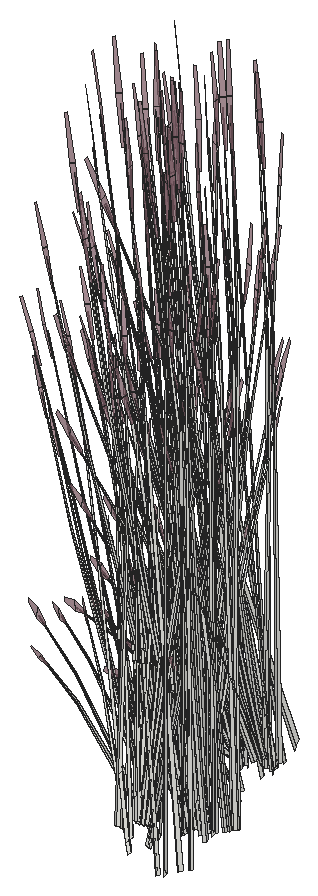
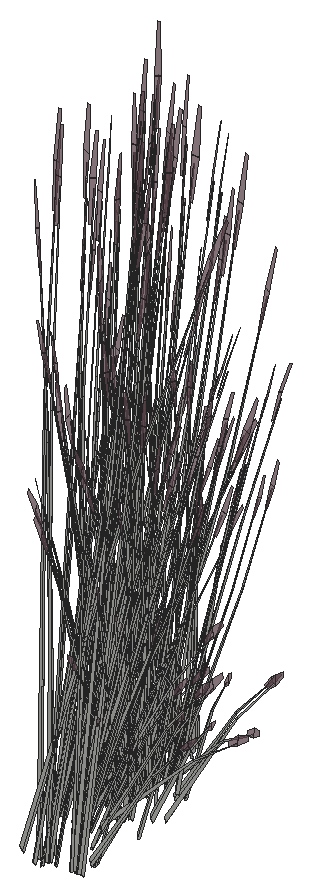
# SketchUp Ruby script. Lengths in inches.
U = 1.inch
M = Sketchup.active_model
def pt(a) = Geom::Point3d.new(a.map { |v| v * U })
def face(e, loops, mat)
  f = e.add_face(loops[0].map { |a| pt(a) })
  loops[1..].each { |l| e.add_face(l.map { |a| pt(a) }).erase! }
  f.material = f.back_material = mat if mat
  f
end
# faces: each face lists its corners as indices into pts; further lists are holes
def faces(e, pts, list, mat = nil) = list.each { |f| face(e, (f[0].is_a?(Array) ? f : [f]).map { |l| l.map { |i| pts[i] } }, mat) }
# xy, xz, yz: faces in a plane at the given z, y or x. An outline is a flat list of corners, or four numbers for a rectangle; further outlines are holes
def ring(l) = l.size == 4 ? [[l[0], l[1]], [l[2], l[1]], [l[2], l[3]], [l[0], l[3]]] : l.each_slice(2).to_a
def flat(e, list, mat, &to3) = list.each { |f| face(e, (f[0].is_a?(Array) ? f : [f]).map { |l| ring(l).map { |u, v| to3.(u, v) } }, mat) }
def xy(e, z, list, mat = nil) = flat(e, list, mat) { |x, y| [x, y, z] }
def xz(e, y, list, mat = nil) = flat(e, list, mat) { |x, z| [x, y, z] }
def yz(e, x, list, mat = nil) = flat(e, list, mat) { |y, z| [x, y, z] }
def lines(e, pts, list) = list.each { |a, b| e.add_line(pt(pts[a]), pt(pts[b])) }
# prism: a flat outline (further loops are holes) pulled along v
def prism(e, loops, v, mat = nil)
  f = face(e, loops, mat); d = Geom::Vector3d.new(v.map { |x| x * U })
  f.pushpull(f.normal.samedirection?(d) ? d.length : -d.length)
end
def box(e, o, s, mat = nil) = prism(e, [[o, [o[0] + s[0], o[1], o[2]], [o[0] + s[0], o[1] + s[1], o[2]], [o[0], o[1] + s[1], o[2]]]], [0, 0, s[2]], mat)
def at(x, y, z, deg = 0) = Geom::Transformation.translation(pt([x, y, z])) * Geom::Transformation.rotation(ORIGIN, Z_AXIS, deg.degrees)
def axes(o, x, y, z) = Geom::Transformation.new([*x, 0, *y, 0, *z, 0, *pt(o).to_a, 1])
def part(name) = M.definitions.add(name)
# library, detail: a bought-in or finely detailed component or shape, given as its bounding box
def library(name, o, s) = part(name).tap { |d| box(d.entities, o, s) }
def detail(e, o, s) = box(e.add_group.entities, o, s)
def put(e, d, t, mat = nil) = e.add_instance(d, t).tap { |i| i.material = mat if mat }
def group(e, t, mat = nil) = e.add_group.tap { |g| g.transformation = t; g.material = mat if mat }.entities
root = M.entities
M.materials.add("LightPink_Translucent").color = [144, 107, 117]
M.materials["LightPink_Translucent"].alpha = 0.75
c1 = part("blade")
p = [[2.15,0.21,22],[0,0.17,0],[0.09,0.45,0],[2.18,0.31,22],[2.29,0.31,22],[0.38,0.45,0],
  [2.48,0.24,33],[2.49,0.24,33],[2.48,0.22,33]]
faces(c1.entities,p,[[0,1,2,3],[4,5,2,3],[6,3,4,7],[8,0,3,6]])
c2 = part("seeds")
p = [[0.3,-0.1,1.38],[-0.01,-0.03,1.59],[-0.01,-0.03,0.03],[0.14,-0.07,-0.07],[0.29,-0.03,3],[0.15,0.01,3.11]]
faces(c2.entities,p,[[0,1,2,3],[1,0,4,5]],"LightPink_Translucent")
c3 = part("blade with seeds")
put(c3.entities,c1,at(0,0,0))
put(c3.entities,c2,axes([2.4,0.25,30.99],[1.5799,-0.05474,1.17369],[-0.12525,1.92788,0.29478],[-0.07173,-0.02425,1.56792]))
put(root,c3,axes([684.71,328.74,393.91],[0.04823,0.05698,1.47228],[-0.23252,0.51221,-0.13912],[-0.23548,0.00371,0.26054]))
put(root,c3,axes([685.2,321.78,393.91],[-0.10624,0.07413,1.45204],[0.00904,0.54162,-0.22964],[-0.24352,0.07044,0.11645]))
put(root,c3,axes([685.25,328.4,393.91],[-0.13998,-0.00403,1.45204],[-0.44565,0.40302,-0.22964],[-0.23779,-0.08235,0.11645]))
put(root,c3,axes([685.625,329.4,394.18],[-0.03484,0.58066,-0.10093],[-0.65957,-0.01587,-0.56021],[-0.25402,-0.04034,0.85122]))
put(root,c3,axes([685.54,321.47,393.76],[-0.54068,-0.15928,-0.29394],[0.1577,-0.46469,0.37948],[-0.21769,0.04261,0.72609]))
put(root,c3,axes([685.2,329.45,393.76],[-0.37017,-0.35748,-0.29394],[0.42268,-0.3384,0.37948],[-0.21476,-0.05149,0.72609]))
put(root,c3,axes([684.02,322.33,393.91],[0.08303,0.01531,1.47228],[0.25685,0.50448,-0.13912],[-0.16996,0.13241,0.26054]))
put(root,c3,axes([685.91,321.71,393.89],[-0.17625,0.51936,-0.42412],[-0.60429,-0.17802,-0.32852],[-0.2433,0.04762,0.81151]))
put(root,c3,axes([684.31,330.3,392.3],[0.41536,-0.04086,0.95334],[-0.26347,0.35999,0.70045],[-0.20525,-0.054,0.20998]))
put(root,c3,axes([685.61,321.68,391.24],[0.0165,0.08998,1.46364],[-0.33262,0.46992,-0.2236],[-0.23626,-0.02369,0.24931]))
put(root,c3,axes([685.14,329.3125,394.23],[0.53728,-0.42137,0.44623],[0.46337,0.44748,0.36794],[-0.25207,-0.07773,0.92337]))
put(root,c3,axes([684.72,323.93,392.3],[0.27113,-0.25877,0.95334],[0.10699,0.40966,0.70045],[-0.19594,0.07335,0.20998]))
put(root,c3,axes([685.67,321.41,393.93],[0.18381,-0.5206,0.39842],[0.60429,0.17802,0.32852],[-0.23764,0.03129,0.82444]))
put(root,c3,axes([685.88,321.26,394.18],[0.32734,0.51701,-0.10093],[-0.58097,0.25407,-0.56021],[-0.24483,0.06821,0.85122]))
put(root,c3,axes([686.62,320.19,394.18],[-0.03484,0.58066,-0.10093],[-0.65957,-0.01587,-0.56021],[-0.25402,-0.04034,0.85122]))
put(root,c3,axes([685.62,321.28,393.93],[-0.23895,-0.38931,0.05337],[0.43573,-0.19055,0.42015],[-0.19208,0.0376,0.64067]))
put(root,c3,axes([686.72,322.35,393.22],[0.1625,-0.17544,1.42242],[0.41029,0.47354,0.11501],[-0.28141,0.21565,0.60807]))
put(root,c3,axes([685.74,322.8125,393.76],[-0.56631,0.0816,-0.29394],[-0.14954,-0.46647,0.37948],[-0.16229,0.12529,0.72609]))
put(root,c3,axes([685.43,324.2,391.24],[0.08727,0.05704,1.46364],[0.14797,0.52853,-0.2236],[-0.19341,0.11271,0.24931]))
put(root,c3,axes([685.39,329.31,393.93],[0.03276,-0.43418,0.05337],[0.49468,0.0119,0.42015],[-0.18949,-0.04543,0.64067]))
put(root,c3,axes([685.31,321.09,392.3],[0.41536,-0.04086,0.95334],[-0.26347,0.35999,0.70045],[-0.20525,-0.054,0.20998]))
put(root,c3,axes([686.91,328.56,394.51],[-0.4342,0.54737,-0.11304],[-0.6288,-0.31535,-0.62743],[-0.21858,-0.15465,0.95337]))
put(root,c3,axes([685.72,329.63,394.19],[0.37017,0.35748,0.29394],[-0.42268,0.3384,-0.37948],[-0.21476,-0.05149,0.72609]))
put(root,c3,axes([685.8125,322.71,393.93],[-0.16135,-0.52549,0.39842],[0.63294,-0.0912,0.32852],[-0.18654,0.12359,0.82444]))
put(root,c3,axes([686.72,329,394.13],[-0.55475,-0.27598,-0.58968],[0.39425,-0.48361,0.07116],[-0.20099,-0.16478,0.83415]))
put(root,c3,axes([686.46,329.02,393.89],[-0.64198,0.13573,-0.42412],[-0.1123,-0.514,-0.32852],[-0.17243,-0.1473,0.81151]))
put(root,c3,axes([685.6875,322.61,393.93],[-0.44663,-0.24013,0.05337],[0.26003,-0.34195,0.42015],[-0.14319,0.11055,0.64067]))
put(root,c3,axes([685.63,328.55,391.24],[-0.06302,0.07522,1.46364],[-0.63686,0.16217,-0.2236],[-0.15385,-0.14752,0.24931]))
put(root,c3,axes([686.6,322.79,393.22],[0.12114,-0.19625,1.42242],[0.50818,0.40613,0.11501],[-0.22925,0.25313,0.60807]))
put(root,c3,axes([687.5,316.97,393.22],[0.1625,-0.17544,1.42242],[0.41029,0.47354,0.11501],[-0.28141,0.21565,0.60807]))
put(root,c3,axes([686.22,318.81,391.24],[0.08727,0.05704,1.46364],[0.14797,0.52853,-0.2236],[-0.19341,0.11271,0.24931]))
put(root,c3,axes([686.11,321.42,394.19],[0.54068,0.15928,0.29394],[-0.1577,0.46469,-0.37948],[-0.21769,0.04261,0.72609]))
put(root,c3,axes([686.21,322.87,393.89],[0.16713,0.52135,-0.42412],[-0.63294,0.0912,-0.32852],[-0.18138,0.14003,0.81151]))
put(root,c3,axes([685.22,323.8,393.91],[-0.01617,0.11299,1.45204],[0.45894,0.39307,-0.22964],[-0.12015,0.18588,0.11645]))
put(root,c3,axes([687.79,322.49,391.71],[-0.67676,-0.09361,-0.51753],[0.14281,-0.57742,-0.13583],[-0.20196,-0.06997,1.14236]))
put(root,c3,axes([685.24,328.84,391.77],[-0.18768,0.46622,-0.03231],[-0.57763,-0.14342,-0.14649],[-0.0877,-0.07626,0.48318]))
put(root,c3,axes([686.74,327.26,393.91],[-0.01214,0.06844,1.47228],[-0.59861,0.24837,-0.13912],[-0.17615,-0.12696,0.26054]))
put(root,c3,axes([686.1,328.25,392.15],[-0.0394,0.18678,1.18691],[-0.57594,0.15636,-0.25526],[-0.13463,-0.24142,0.50747]))
put(root,c3,axes([687.38,317.4,393.22],[0.12114,-0.19625,1.42242],[0.50818,0.40613,0.11501],[-0.22925,0.25313,0.60807]))
put(root,c3,axes([686.29,328.73,393.22],[0.14872,0.18332,1.42242],[-0.6872,0.15433,0.11501],[-0.15531,-0.28779,0.60807]))
put(root,c3,axes([686.9,323.59,391.67],[-0.60889,-0.28548,-0.4121],[0.36394,-0.51192,0],[-0.13868,-0.06502,1.30728]))
put(root,c3,axes([685.91,322.49,394.18],[0.60181,0.31483,-0.10093],[-0.34671,0.45593,-0.56021],[-0.17003,0.15849,0.85122]))
put(root,c3,axes([686.53,328.64,393.76],[-0.10048,-0.4599,-0.29394],[0.5744,-0.12144,0.37948],[-0.15428,-0.13179,0.72609]))
put(root,c3,axes([687.27,323.93,391.97],[-0.40676,0.57214,0],[-0.68052,-0.31907,-0.42834],[-0.15499,-0.07267,1.3588]))
put(root,c3,axes([684.93,330.96,391.97],[-0.81352,0,0],[0,-0.63814,-0.42834],[0,-0.14534,1.3588]))
put(root,c3,axes([686.99,317.48,393.89],[0.16713,0.52135,-0.42412],[-0.63294,0.0912,-0.32852],[-0.18138,0.14003,0.81151]))
put(root,c3,axes([686,318.42,393.91],[-0.01617,0.11299,1.45204],[0.45894,0.39307,-0.22964],[-0.12015,0.18588,0.11645]))
put(root,c3,axes([684.92,323.86,394.6875],[0.5741,0.15241,-0.05385],[-0.1766,0.46909,-0.24415],[-0.0939,0.07122,0.8053]))
put(root,c3,axes([686.87,329.01,394.19],[0.10048,0.4599,0.29394],[-0.5744,0.12144,-0.37948],[-0.15428,-0.13179,0.72609]))
put(root,c3,axes([686.2,322.54,394.19],[0.56631,-0.0816,0.29394],[0.14954,0.46647,-0.37948],[-0.16229,0.12529,0.72609]))
put(root,c3,axes([685.56,330.8,391.93],[-0.60515,0.48003,0.25528],[-0.60552,-0.47498,-0.30288],[-0.02113,-0.13632,1.36855]))
put(root,c3,axes([686.53,324.76,392.15],[0.2053,-0.09007,1.18691],[0.50689,0.27159,-0.25526],[-0.15087,0.235,0.50747]))
put(root,c3,axes([688.05,332.125,392.76],[0.56221,0.23024,1.25546],[-0.55078,0.49601,0.49647],[-0.2467,-0.29398,1.05249]))
put(root,c3,axes([685.9,327.95,392.3],[0.33937,0.19872,0.95334],[-0.49424,0.11946,0.70045],[-0.10575,-0.15273,0.20998]))
put(root,c3,axes([687.14,331.52,391.83],[-0.39083,-0.47924,-0.37133],[0.59199,-0.33747,0.17871],[-0.12647,-0.0593,1.19224]))
put(root,c3,axes([686.69,317.11,394.18],[0.60181,0.31483,-0.10093],[-0.34671,0.45593,-0.56021],[-0.17003,0.15849,0.85122]))
put(root,c3,axes([688.55,322.58,392.21],[-0.65687,0.37907,-0.24149],[-0.43681,-0.53562,-0.41502],[-0.16207,-0.0544,1.32557]))
put(root,c3,axes([686.61,328.47,394.23],[0.72473,-0.14676,0.44623],[0.12578,0.57568,0.36794],[-0.17045,-0.16967,0.92337]))
put(root,c3,axes([686.74,323.77,393.93],[-0.46327,-0.38957,0.39842],[0.49199,-0.33598,0.32852],[-0.08546,0.18277,0.82444]))
put(root,c3,axes([687.07,323.37,391.68],[-0.15283,-0.49751,-0.25712],[0.60696,-0.14127,0.25712],[-0.12236,-0.05737,1.15348]))
put(root,c3,axes([686.57,323.74,393.93],[-0.53464,-0.0266,0.05337],[0.01466,-0.40172,0.42015],[-0.05594,0.15388,0.64067]))
put(root,c3,axes([686.78,328.59,393.93],[0.29569,-0.36271,0.05337],[0.42107,0.21117,0.42015],[-0.13613,-0.11629,0.64067]))
put(root,c3,axes([686.74,323.89,393.76],[-0.4402,0.30062,-0.29394],[-0.41671,-0.34326,0.37948],[-0.0634,0.1744,0.72609]))
put(root,c3,axes([687.31,319.37,392.15],[0.2053,-0.09007,1.18691],[0.50689,0.27159,-0.25526],[-0.15087,0.235,0.50747]))
put(root,c3,axes([687.2,331.8,392.02],[0.17244,-0.67657,-0.19446],[0.81759,0.11793,0.42555],[-0.14286,-0.09343,1.29846]))
put(root,c3,axes([688.99,322.99,391.71],[-0.43821,0.42916,-0.51753],[-0.54436,-0.38915,-0.13583],[-0.1756,0.10706,1.14236]))
put(root,c3,axes([685.17,324.96,393.91],[0.07381,-0.03447,1.47228],[0.61004,0.22929,-0.13912],[-0.01434,0.19091,0.26054]))
put(root,c3,axes([687.42,327.52,393.91],[-0.09951,-0.08005,1.45204],[-0.66407,0.05075,-0.22964],[-0.10598,-0.19148,0.11645]))
put(root,c3,axes([685.11,330.53,391.67],[0,-0.57097,-0.4121],[0.72788,0,0],[0,-0.13004,1.30728]))
put(root,c3,axes([685.42,331.0625,392.06],[0,0.57097,0.4121],[-0.72788,0,0],[0,-0.13004,1.30728]))
put(root,c3,axes([689.29,322.75,392.05],[-0.63528,-0.45956,-0.20909],[0.53456,-0.51604,0.45758],[-0.17107,0.05376,1.39619]))
put(root,c3,axes([688.14,322.31,391.83],[-0.39083,-0.47924,-0.37133],[0.59199,-0.33747,0.17871],[-0.12647,-0.0593,1.19224]))
put(root,c3,axes([687.52,318.39,393.93],[-0.46327,-0.38957,0.39842],[0.49199,-0.33598,0.32852],[-0.08546,0.18277,0.82444]))
put(root,c3,axes([687.03,323.57,394.43],[-0.01693,0.52814,-0.65454],[-0.71285,-0.03547,0.07899],[-0.07523,0.22375,0.92591]))
put(root,c3,axes([687.35,318.35,393.93],[-0.53464,-0.0266,0.05337],[0.01466,-0.40172,0.42015],[-0.05594,0.15388,0.64067]))
put(root,c3,axes([687.02,325.06,392.3],[-0.01684,-0.3395,0.95334],[0.42072,0.24214,0.70045],[-0.08274,0.16182,0.20998]))
put(root,c3,axes([687.01,331.19,392.21],[-0.73268,-0.27244,-0.24149],[0.35279,-0.57501,-0.41502],[-0.02303,-0.14118,1.32557]))
put(root,c3,axes([688.97,322.65,391.83],[-0.70648,0.03525,-0.37133],[-0.06389,-0.58508,0.17871],[-0.12647,0.0593,1.19224]))
put(root,c3,axes([687.52,318.51,393.76],[-0.4402,0.30062,-0.29394],[-0.41671,-0.34326,0.37948],[-0.0634,0.1744,0.72609]))
put(root,c3,axes([689.77,317.61,391.71],[-0.43821,0.42916,-0.51753],[-0.54436,-0.38915,-0.13583],[-0.1756,0.10706,1.14236]))
put(root,c3,axes([687.62,323.63,392.06],[0.60889,0.28548,0.4121],[-0.36394,0.51192,0],[-0.13868,-0.06502,1.30728]))
put(root,c3,axes([686.68,330.61,391.74],[-0.26718,-0.5855,-0.57963],[0.76964,-0.21087,-0.15213],[-0.02953,-0.19827,1.27944]))
put(root,c3,axes([685.95,319.58,393.91],[0.07381,-0.03447,1.47228],[0.61004,0.22929,-0.13912],[-0.01434,0.19091,0.26054]))
put(root,c3,axes([688.43,328.75,394.18],[-0.63664,0.26583,-0.10093],[-0.31286,-0.47181,-0.56021],[-0.084,-0.19882,0.85122]))
put(root,c3,axes([686.79,324.32,392.79],[0.01429,-0.29475,1.28107],[0.64291,0.15569,0.17703],[-0.0557,0.31414,0.60492]))
put(root,c3,axes([687.89,328.78,393.89],[-0.63954,-0.14313,-0.42412],[0.21921,-0.49074,-0.32852],[-0.05864,-0.19758,0.81151]))
put(root,c3,axes([688.49,322.74,392.17],[-0.12551,0.50956,0.12018],[-0.6132,-0.08845,-0.34318],[-0.1116,-0.05232,1.05198]))
put(root,c3,axes([685.42,330.54,391.68],[0.45414,-0.35624,-0.25712],[0.45414,0.35624,0.25712],[0,-0.11474,1.15348]))
put(root,c3,axes([687.47,328.24,391.77],[-0.44958,0.32756,-0.03231],[-0.41194,-0.35875,-0.14649],[-0.029,-0.10165,0.48318]))
put(root,c3,axes([689.71,324.16,391.67],[-0.60889,0.28548,-0.4121],[-0.36394,-0.51192,0],[-0.13868,0.06502,1.30728]))
put(root,c3,axes([686.42,321.85,392.06],[0,0.57097,0.4121],[-0.72788,0,0],[0,-0.13004,1.30728]))
put(root,c3,axes([689.75,324.01,391.82],[-0.40169,-0.57414,-0.04268],[0.68052,-0.31907,0.42834],[-0.16769,0.05466,1.35813]))
put(root,c3,axes([687.81,318.1875,394.43],[-0.01693,0.52814,-0.65454],[-0.71285,-0.03547,0.07899],[-0.07523,0.22375,0.92591]))
put(root,c3,axes([687.8,319.67,392.3],[-0.01684,-0.3395,0.95334],[0.42072,0.24214,0.70045],[-0.08274,0.16182,0.20998]))
put(root,c3,axes([687.17,323.75,394.15],[0.46573,0.38364,-0.47077],[-0.49199,0.33598,-0.36465],[-0.07086,0.19492,0.90078]))
put(root,c3,axes([687.08,331.35,392.26],[-0.31565,0.51449,0.37133],[-0.65588,-0.24761,-0.17871],[0,-0.1186,1.19224]))
put(root,c3,axes([688.12,328.87,394.13],[-0.31051,-0.46426,-0.58968],[0.63919,-0.25873,0.07116],[-0.07261,-0.22432,0.83415]))
put(root,c3,axes([689.57,323.9375,391.68],[-0.60696,-0.14127,-0.25712],[0.15283,-0.49751,0.25712],[-0.12236,0.05737,1.15348]))
put(root,c3,axes([686.97,323.47,394.19],[0.4402,-0.30062,0.29394],[0.41671,0.34326,-0.37948],[-0.0634,0.1744,0.72609]))
put(root,c3,axes([689.92,321.81,392.36],[-0.01777,-0.53759,1.17256],[0.80434,0.13935,0.49647],[-0.19024,0.29416,1.1068]))
put(root,c3,axes([687.58,318.93,392.79],[0.01429,-0.29475,1.28107],[0.64291,0.15569,0.17703],[-0.0557,0.31414,0.60492]))
put(root,c3,axes([686.6875,323.55,394.48],[0.71502,0.02829,-0.11203],[-0.01954,0.53563,-0.62183],[-0.04967,0.20629,0.94486]))
put(root,c3,axes([686.67,324.33,392.34],[0.59102,-0.10111,0.05401],[0.13587,0.40735,-0.71633],[-0.03747,0.2062,0.64209]))
put(root,c3,axes([688.24,328.9375,394.19],[-0.19614,0.43908,0.29394],[-0.57222,-0.12807,-0.37948],[-0.05247,-0.17678,0.72609]))
put(root,c3,axes([689.46,322.49,392.21],[0.07581,0.65151,-0.24149],[-0.7896,0.03939,-0.41502],[-0.13904,0.08678,1.32557]))
put(root,c3,axes([690.5,318.78,391.67],[-0.60889,0.28548,-0.4121],[-0.36394,-0.51192,0],[-0.13868,0.06502,1.30728]))
put(root,c3,axes([687.7,323.2,393.22],[-0.01592,-0.21915,1.42242],[0.69015,0.14538,0.11501],[-0.04269,0.3123,0.60807]))
put(root,c3,axes([687.96,318.36,394.15],[0.46573,0.38364,-0.47077],[-0.49199,0.33598,-0.36465],[-0.07086,0.19492,0.90078]))
put(root,c3,axes([688.29,322.26,391.96],[0.82229,0.1203,0.37976],[-0.16734,0.67942,0.14902],[-0.12017,-0.06561,1.31851]))
put(root,c3,axes([687.75,318.08,394.19],[0.4402,-0.30062,0.29394],[0.41671,0.34326,-0.37948],[-0.0634,0.1744,0.72609]))
put(root,c3,axes([690.7,316.42,392.36],[-0.01777,-0.53759,1.17256],[0.80434,0.13935,0.49647],[-0.19024,0.29416,1.1068]))
put(root,c3,axes([688.08,322.13,392.26],[-0.31565,0.51449,0.37133],[-0.65588,-0.24761,-0.17871],[0,-0.1186,1.19224]))
put(root,c3,axes([687.58,327.84,391.24],[-0.10912,0.02057,1.46364],[-0.60346,-0.23156,-0.2236],[0.01013,-0.19315,0.24931]))
put(root,c3,axes([687.47,318.16,394.48],[0.71502,0.02829,-0.11203],[-0.01954,0.53563,-0.62183],[-0.04967,0.20629,0.94486]))
put(root,c3,axes([688.18,328.48,393.76],[0.19614,-0.43908,-0.29394],[0.57222,0.12807,0.37948],[-0.05247,-0.17678,0.72609]))
put(root,c3,axes([687.22,330.85,391.96],[0.28286,0.63846,0.37976],[-0.80821,0.22202,0.14902],[0.00988,-0.11732,1.31851]))
put(root,c3,axes([687.45,318.9375,392.34],[0.59102,-0.10111,0.05401],[0.13587,0.40735,-0.71633],[-0.03747,0.2062,0.64209]))
put(root,c3,axes([687.09,330.76,391.83],[0.31565,-0.51449,-0.37133],[0.65588,0.24761,0.17871],[0,-0.1186,1.19224]))
put(root,c3,axes([687.85,323.34,392.05],[0.6991,-0.15154,0.14643],[0.17263,0.56398,0.29122],[-0.06235,-0.08217,1.33138]))
put(root,c3,axes([688.49,317.8125,393.22],[-0.01592,-0.21915,1.42242],[0.69015,0.14538,0.11501],[-0.04269,0.3123,0.60807]))
put(root,c3,axes([688.75,323.43,391.82],[-0.65588,-0.25634,0],[0.31565,-0.53263,0],[0,0,1.35047]))
put(root,c3,axes([690.26,324.07,391.97],[0.40676,0.57214,0],[-0.68052,0.31907,-0.42834],[-0.15499,0.07267,1.3588]))
put(root,c3,axes([688.19,324.32,394.2],[-0.64106,-0.14927,0.44225],[0.21921,-0.49074,0.36465],[0.03852,0.19299,0.91512]))
put(root,c3,axes([688.02,324.36,393.93],[-0.47939,0.19405,0.05337],[-0.23464,-0.35385,0.42015],[0.0463,0.15598,0.64067]))
put(root,c3,axes([689.93,323.375,392.05],[0.18794,-0.56744,0.14643],[0.68774,0.16058,0.29122],[-0.1188,0.00276,1.33138]))
put(root,c3,axes([689.61,322.62,392.17],[0.48065,0.34305,0.12018],[-0.40092,0.38703,-0.34318],[-0.1116,0.05232,1.05198]))
put(root,c3,axes([689.4375,322.2,391.91],[-0.60515,-0.49144,-0.05089],[0.60552,-0.49174,0],[-0.02113,-0.01716,1.45724]))
put(root,c3,axes([688.42,328.54,393.93],[0.47939,-0.19405,0.05337],[0.23464,0.35385,0.42015],[-0.0463,-0.15598,0.64067]))
put(root,c3,axes([689.6,322.37,392.26],[0.70648,-0.03525,0.37133],[0.06389,0.58508,-0.17871],[-0.12647,0.0593,1.19224]))
put(root,c3,axes([688.25,328.58,393.93],[0.64106,0.14927,0.39842],[-0.21921,0.49074,0.32852],[-0.03852,-0.19299,0.82444]))
put(root,c3,axes([689.77,323.71,391.93],[0.81449,0.18558,0.25528],[-0.20377,0.66335,-0.30288],[-0.13481,0.08302,1.36855]))
put(root,c3,axes([687.48,331.02,392.02],[0.73304,0.27674,0.19974],[-0.35279,0.57501,0.41502],[0,-0.13255,1.3325]))
put(root,c3,axes([687.25,330.63,392.26],[-0.70648,0.03525,0.37133],[-0.06389,-0.58508,-0.17871],[0.12647,-0.0593,1.19224]))
put(root,c3,axes([690.12,323.68,392.06],[0.60889,-0.28548,0.4121],[0.36394,0.51192,0],[-0.13868,0.06502,1.30728]))
put(root,c3,axes([688.22,321.63,391.96],[0.28286,0.63846,0.37976],[-0.80821,0.22202,0.14902],[0.00988,-0.11732,1.31851]))
put(root,c3,axes([691.05,318.6875,391.97],[0.40676,0.57214,0],[-0.68052,0.31907,-0.42834],[-0.15499,0.07267,1.3588]))
